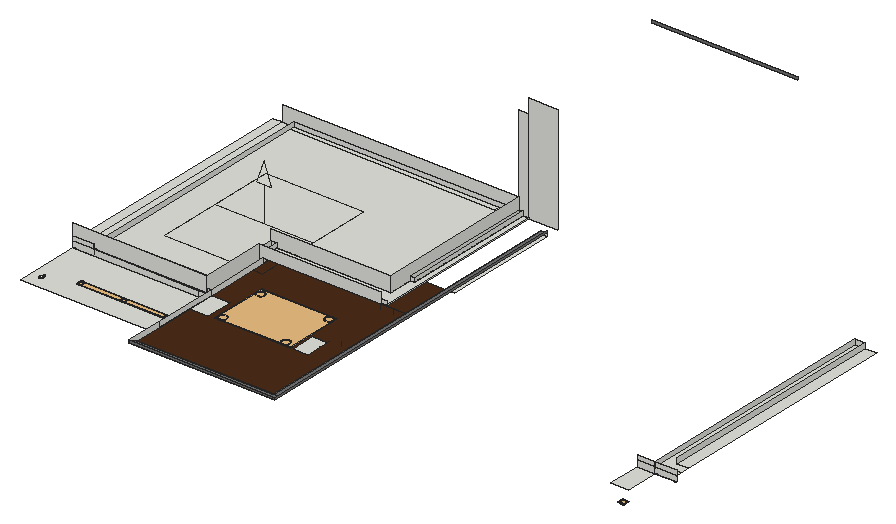
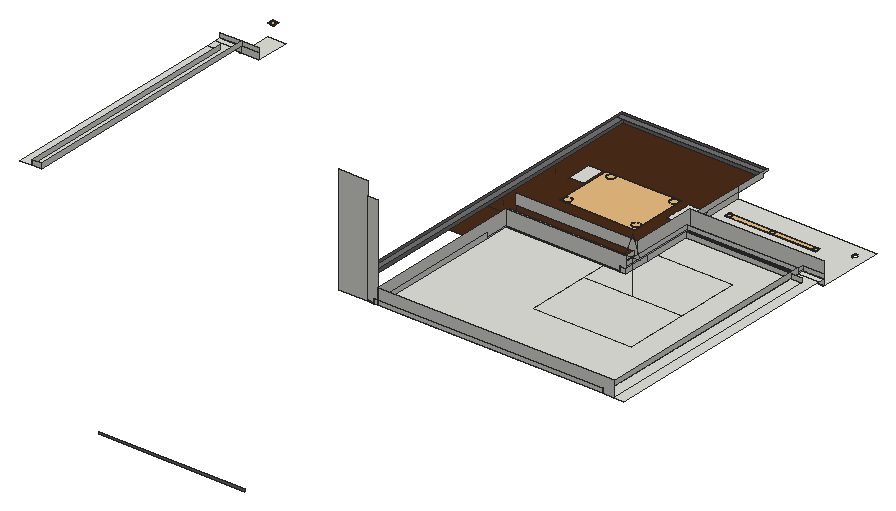
# SketchUp Ruby script. Lengths in inches.
U = 1.inch
M = Sketchup.active_model
def pt(a) = Geom::Point3d.new(a.map { |v| v * U })
def face(e, loops, mat)
  f = e.add_face(loops[0].map { |a| pt(a) })
  loops[1..].each { |l| e.add_face(l.map { |a| pt(a) }).erase! }
  f.material = f.back_material = mat if mat
  f
end
# faces: each face lists its corners as indices into pts; further lists are holes
def faces(e, pts, list, mat = nil) = list.each { |f| face(e, (f[0].is_a?(Array) ? f : [f]).map { |l| l.map { |i| pts[i] } }, mat) }
# xy, xz, yz: faces in a plane at the given z, y or x. An outline is a flat list of corners, or four numbers for a rectangle; further outlines are holes
def ring(l) = l.size == 4 ? [[l[0], l[1]], [l[2], l[1]], [l[2], l[3]], [l[0], l[3]]] : l.each_slice(2).to_a
def flat(e, list, mat, &to3) = list.each { |f| face(e, (f[0].is_a?(Array) ? f : [f]).map { |l| ring(l).map { |u, v| to3.(u, v) } }, mat) }
def xy(e, z, list, mat = nil) = flat(e, list, mat) { |x, y| [x, y, z] }
def xz(e, y, list, mat = nil) = flat(e, list, mat) { |x, z| [x, y, z] }
def yz(e, x, list, mat = nil) = flat(e, list, mat) { |y, z| [x, y, z] }
def lines(e, pts, list) = list.each { |a, b| e.add_line(pt(pts[a]), pt(pts[b])) }
# prism: a flat outline (further loops are holes) pulled along v
def prism(e, loops, v, mat = nil)
  f = face(e, loops, mat); d = Geom::Vector3d.new(v.map { |x| x * U })
  f.pushpull(f.normal.samedirection?(d) ? d.length : -d.length)
end
def box(e, o, s, mat = nil) = prism(e, [[o, [o[0] + s[0], o[1], o[2]], [o[0] + s[0], o[1] + s[1], o[2]], [o[0], o[1] + s[1], o[2]]]], [0, 0, s[2]], mat)
def at(x, y, z, deg = 0) = Geom::Transformation.translation(pt([x, y, z])) * Geom::Transformation.rotation(ORIGIN, Z_AXIS, deg.degrees)
def axes(o, x, y, z) = Geom::Transformation.new([*x, 0, *y, 0, *z, 0, *pt(o).to_a, 1])
def part(name) = M.definitions.add(name)
# library, detail: a bought-in or finely detailed component or shape, given as its bounding box
def library(name, o, s) = part(name).tap { |d| box(d.entities, o, s) }
def detail(e, o, s) = box(e.add_group.entities, o, s)
def put(e, d, t, mat = nil) = e.add_instance(d, t).tap { |i| i.material = mat if mat }
def group(e, t, mat = nil) = e.add_group.tap { |g| g.transformation = t; g.material = mat if mat }.entities
root = M.entities
M.materials.add("[Color M05]").color = [114, 114, 114]
M.materials.add("[Wood Veneer 01]").color = [76, 44, 23]
c1 = library("Group\#26",[-0.5,-0.5,-0.1],[9.125,9.125,0.2])
c2 = library("Group\#20",[-0.5,-0.5,-0.1],[139.5,7.875,0.2])
c3 = library("Group\#21",[-0.5,-0.5,-0.1],[115.36,88.99,0.2])
c4 = part("Group266\#1")
p = [[0,0,0],[0,0,-53.16],[-11.52,0,-53.16],[75.01,-97.09,0],[-75.01,-97.09,0],[75.01,97.09,0],
  [75.01,0,0],[-75.01,97.09,0],[11.52,0,-53.16],[-75.01,0,0],[0,0,-86.05]]
lines(c4.entities,p,[[0,1],[1,2],[3,4],[5,6],[7,5],[1,8],[9,0],[0,6],[8,10],[4,9],[6,3],[2,10],
  [9,7]])
c5 = part("Rectangle Light\#1")
put(c5.entities,c4,at(0,0,0))
xy(root,104.9375,[[[1172.33,538.49,1384.3,638.99],[1186.89,556.14,1187.94,556.28,1188.92,556.69,1189.77,557.33,1190.41,558.17,1190.82,559.15,1190.96,560.2,1190.82,561.26,1190.41,562.23,1189.77,563.08,1188.92,563.72,1187.94,564.13,1186.89,564.27,1185.84,564.13,1184.86,563.72,1184.02,563.08,1183.375,562.23,1182.97,561.26,1182.83,560.2,1182.97,559.15,1183.375,558.17,1184.02,557.33,1184.86,556.69,1185.84,556.28],[1234.95,572.82,1235.84,572.9375,1236.67,573.28,1237.38,573.83,1237.93,574.54,1238.27,575.37,1238.39,576.26,1238.27,577.15,1237.93,577.98,1237.38,578.6875,1236.67,579.23,1235.84,579.58,1234.95,579.69,1234.06,579.58,1233.23,579.23,1232.52,578.6875,1231.97,577.98,1231.63,577.15,1231.51,576.26,1231.63,575.37,1231.97,574.54,1232.52,573.83,1233.23,573.28,1234.06,572.9375],[1300.76,572.82,1301.65,572.9375,1302.48,573.28,1303.19,573.83,1303.74,574.54,1304.08,575.37,1304.2,576.26,1304.08,577.15,1303.74,577.98,1303.19,578.6875,1302.48,579.23,1301.65,579.58,1300.76,579.69,1299.87,579.58,1299.04,579.23,1298.33,578.6875,1297.79,577.98,1297.44,577.15,1297.32,576.26,1297.44,575.37,1297.79,574.54,1298.33,573.83,1299.04,573.28,1299.87,572.9375],[1366.57,572.82,1367.46,572.9375,1368.29,573.28,1369.01,573.83,1369.55,574.54,1369.9,575.37,1370.01,576.26,1369.9,577.15,1369.55,577.98,1369.01,578.6875,1368.29,579.23,1367.46,579.58,1366.57,579.69,1365.69,579.58,1364.86,579.23,1364.14,578.6875,1363.6,577.98,1363.25,577.15,1363.14,576.26,1363.25,575.37,1363.6,574.54,1364.14,573.83,1364.86,573.28,1365.69,572.9375]]])
xy(root,109.5,[[2037.92,586.4375,2064.92,636.6875]])
xy(root,113.8125,[[1384.3,597.99,1411.73,638.93],[1542.45,597.99,1563.95,635.56],[1172.33,638.99,1204.64,648.22],[1204.64,638.99,1365.47,648.22],[1172.33,648.22,1204.64,648.22,1204.64,662.52,1187.0625,662.52,1187.0625,1021.31,1172.33,1021.31],
  [1187.0625,662.52,1204.64,1021.31],[1204.64,662.52,1204.64,1013.93,1548.25,1013.93,1548.25,776.62,1364.27,776.62,1364.27,662.52],[1554.73,749.87,1563.95,1021.31],[1597.39,824.85,1607.7,1001.66],[1204.64,1013.93,1517.39,1021.31],
  [1517.39,1013.93,1548.25,1021.31]])
xy(root,113.8125,[[[1384.3,491.12,1384.3,597.99,1411.73,597.99,1411.73,638.93,1384.3,638.93,1384.3,749.87,1597.39,749.87,1597.39,491.12],[1542.45,597.99,1563.95,635.56],[1525.93,598.1875,1527.48,598.39,1528.93,598.99,1530.17,599.94,1531.13,601.1875,1531.73,602.63,1531.93,604.1875,1531.73,605.74,1531.13,607.1875,1530.17,608.43,1528.93,609.38,1527.48,609.98,1525.93,610.1875,1524.38,609.98,1522.93,609.38,1521.6875,608.43,1520.74,607.1875,1520.14,605.74,1519.93,604.1875,1520.14,602.63,1520.74,601.1875,1521.6875,599.94,1522.93,598.99,1524.38,598.39],[1429.12,670.9375,1430.67,671.14,1432.12,671.74,1433.36,672.69,1434.32,673.9375,1434.92,675.38,1435.12,676.9375,1434.92,678.49,1434.32,679.9375,1433.36,681.18,1432.12,682.13,1430.67,682.73,1429.12,682.9375,1427.57,682.73,1426.12,682.13,1424.875,681.18,1423.92,679.9375,1423.32,678.49,1423.12,676.9375,1423.32,675.38,1423.92,673.9375,1424.875,672.69,1426.12,671.74,1427.57,671.14],[1429.12,598.1875,1430.67,598.39,1432.12,598.99,1433.36,599.94,1434.32,601.1875,1434.92,602.63,1435.12,604.1875,1434.92,605.74,1434.32,607.1875,1433.36,608.43,1432.12,609.38,1430.67,609.98,1429.12,610.1875,1427.57,609.98,1426.12,609.38,1424.875,608.43,1423.92,607.1875,1423.32,605.74,1423.12,604.1875,1423.32,602.63,1423.92,601.1875,1424.875,599.94,1426.12,598.99,1427.57,598.39],[1531.48,674.17,1533.03,674.38,1534.48,674.98,1535.72,675.93,1536.68,677.17,1537.28,678.62,1537.48,680.17,1537.28,681.73,1536.68,683.17,1535.72,684.42,1534.48,685.37,1533.03,685.97,1531.48,686.17,1529.93,685.97,1528.48,685.37,1527.24,684.42,1526.28,683.17,1525.6875,681.73,1525.48,680.17,1525.6875,678.62,1526.28,677.17,1527.24,675.93,1528.48,674.98,1529.93,674.38]],[1563.95,749.87,1597.39,824.85]],"[Wood Veneer 01]")
xy(root,115.0625,[[1204.64,638.99,1376.89,638.99,1376.89,738.06,1384.3,738.06,1384.3,749.87,1563.95,749.87,1563.95,1021.31,1554.73,1021.31,1554.73,813.85,1548.25,813.85,1548.25,776.62,1373.95,776.62,1373.95,648.22,1204.64,648.22]])
xy(root,118.1875,[[1384.3,481.81,1607.7,491.12],[1597.39,491.12,1607.7,1001.66]],"[Color M05]")
xy(root,118.5,[[2064.92,636.6875,2097.23,645.91],[2064.92,645.91,2097.23,645.91,2097.23,660.21,2079.65,660.21,2079.65,1019,2064.92,1019],[2079.65,660.21,2097.23,1019]])
xz(root,481.81,[[1384.3,118.1875,1607.7,121.3125]],"[Color M05]")
xz(root,491.12,[[1384.3,113.8125,1597.39,118.1875]],"[Color M05]")
xz(root,636.6875,[[2037.92,109.5,2064.92,118.5],[2064.92,109.5,2097.23,109.625],[2064.92,109.625,2097.23,118.5],[2037.92,118.5,2064.92,126],[2064.92,118.5,2097.23,126]])
xz(root,638.99,[[1172.33,104.8125,1204.64,104.9375],[1172.33,104.9375,1204.64,113.8125],[1204.64,104.9375,1365.47,113.8125],[1365.47,104.9375,1384.3,113.8125],[1172.33,113.8125,1204.64,121.3125],
  [1204.64,113.8125,1376.89,115.0625],[1376.89,113.8125,1384.3,121.3125],[1204.64,115.0625,1376.89,115.0625,1376.89,138.1875,1172.33,138.1875,1172.33,121.3125,1204.64,121.3125]])
xz(root,648.22,[[1204.64,113.8125,1373.95,115.0625],[1204.64,115.0625,1373.95,121.3125]])
xz(root,662.52,[[1187.0625,113.8125,1364.27,121.3125]])
xz(root,738.06,[[1376.89,113.8125,1384.3,115.0625],[1376.89,115.0625,1384.3,115.0625,1384.3,121.3125,1563.95,121.3125,1563.95,138.1875,1376.89,138.1875]])
xz(root,749.87,[[1384.3,113.8125,1554.73,115.0625],[1554.73,113.8125,1563.95,115.0625],[1384.3,115.0625,1563.95,121.3125]])
xz(root,776.62,[[1364.27,113.8125,1373.95,121.3125],[1373.95,113.8125,1548.25,115.0625],[1373.95,115.0625,1548.25,115.0625,1548.25,138.1875,1364.27,138.1875,1364.27,121.3125,1373.95,121.3125]])
xz(root,813.85,[[1548.25,113.8125,1554.73,115.0625],[1548.25,115.0625,1554.73,121.3125]])
xz(root,1001.66,[[1597.39,113.8125,1607.7,118.1875]])
xz(root,1019,[[2064.92,118.5,2079.65,126]])
xz(root,1021.31,[[1187.0625,113.8125,1187.0625,138.1875,1548.25,138.1875,1548.25,121.3125,1204.64,121.3125,1204.64,113.8125],[1204.64,113.8125,1548.25,121.3125],[1548.25,113.8125,1554.73,121.3125],[1554.73,113.8125,1563.95,115.0625],[1563.95,113.8125,1607.7,279.25],
  [1554.73,115.0625,1554.73,121.3125,1548.25,121.3125,1548.25,258.1875,1563.95,258.1875,1563.95,115.0625]])
xz(root,1481.16,[[1384.3,118.1875,1607.7,121.3125]],"[Color M05]")
yz(root,1204.64,[[638.99,113.8125,648.22,115.0625],[648.22,113.8125,1021.31,121.3125],[638.99,115.0625,648.22,121.3125]])
yz(root,1364.27,[[662.52,113.8125,738.06,121.3125],[738.06,113.8125,776.62,121.3125]])
yz(root,1373.95,[[648.22,113.8125,776.62,115.0625],[648.22,115.0625,776.62,121.3125]])
yz(root,1376.89,[[638.99,113.8125,738.06,115.0625],[638.99,115.0625,738.06,138.1875]])
yz(root,1384.3,[[538.49,104.9375,597.99,113.8125],[597.99,104.9375,638.93,113.8125],[638.93,104.9375,638.99,113.8125],[491.12,113.8125,491.12,118.1875,481.81,118.1875,481.81,121.3125,538.49,121.3125,538.49,113.8125],[538.49,113.8125,638.99,121.3125],
  [638.99,113.8125,738.06,121.3125],[738.06,113.8125,749.87,115.0625],[738.06,115.0625,749.87,121.3125]])
yz(root,1548.25,[[776.62,113.8125,813.85,115.0625],[813.85,113.8125,1021.31,121.3125],[776.62,115.0625,813.85,115.0625,813.85,121.3125,1021.31,121.3125,1021.31,138.1875,776.62,138.1875]])
yz(root,1554.73,[[813.85,113.8125,1021.31,115.0625],[813.85,115.0625,1021.31,121.3125]])
yz(root,1563.95,[[749.87,113.8125,1021.31,115.0625]])
yz(root,1597.39,[[491.12,113.8125,1001.66,118.1875]],"[Color M05]")
yz(root,1607.7,[[481.81,118.1875,1001.66,121.3125]],"[Color M05]")
yz(root,2064.92,[[636.6875,118.5,1019,126]])
yz(root,2079.65,[[660.21,118.5,1019,126]])
p = [[1187.94,556.28,104.9375],[1186.89,556.14,104.9375],[1186.89,556.14,105.875],[1187.94,556.28,105.875],[1188.92,556.69,104.9375],[1188.92,556.69,105.875],
  [1189.77,557.33,104.9375],[1189.77,557.33,105.875],[1190.41,558.17,104.9375],[1190.41,558.17,105.875],[1190.82,559.15,104.9375],[1190.82,559.15,105.875],
  [1190.96,560.2,104.9375],[1190.96,560.2,105.875],[1190.82,561.26,104.9375],[1190.82,561.26,105.875],[1190.41,562.23,104.9375],[1190.41,562.23,105.875],
  [1189.77,563.08,104.9375],[1189.77,563.08,105.875],[1188.92,563.72,104.9375],[1188.92,563.72,105.875],[1187.94,564.13,104.9375],[1187.94,564.13,105.875],
  [1186.89,564.27,104.9375],[1186.89,564.27,105.875],[1234.95,572.82,104.9375],[1234.06,572.9375,104.9375],[1234.06,572.9375,105.375],[1234.95,572.82,105.375],
  [1235.84,572.9375,104.9375],[1235.84,572.9375,105.375],[1300.76,572.82,104.9375],[1299.87,572.9375,104.9375],[1299.87,572.9375,105.375],[1300.76,572.82,105.375],
  [1301.65,572.9375,104.9375],[1301.65,572.9375,105.375],[1366.57,572.82,104.9375],[1365.69,572.9375,104.9375],[1365.69,572.9375,105.375],[1366.57,572.82,105.375],
  [1367.46,572.9375,104.9375],[1367.46,572.9375,105.375],[1233.23,573.28,104.9375],[1233.23,573.28,105.375],[1236.67,573.28,104.9375],[1236.67,573.28,105.375],
  [1299.04,573.28,104.9375],[1299.04,573.28,105.375],[1302.48,573.28,104.9375],[1302.48,573.28,105.375],[1364.86,573.28,104.9375],[1364.86,573.28,105.375],
  [1368.29,573.28,104.9375],[1368.29,573.28,105.375],[1232.52,573.83,104.9375],[1232.52,573.83,105.375],[1237.38,573.83,104.9375],[1237.38,573.83,105.375],
  [1298.33,573.83,104.9375],[1298.33,573.83,105.375],[1303.19,573.83,104.9375],[1303.19,573.83,105.375],[1364.14,573.83,104.9375],[1364.14,573.83,105.375],
  [1369.01,573.83,104.9375],[1369.01,573.83,105.375],[1231.97,574.54,104.9375],[1231.97,574.54,105.375],[1237.93,574.54,104.9375],[1237.93,574.54,105.375],
  [1297.79,574.54,104.9375],[1297.79,574.54,105.375],[1303.74,574.54,104.9375],[1303.74,574.54,105.375],[1363.6,574.54,104.9375],[1363.6,574.54,105.375],
  [1369.55,574.54,104.9375],[1369.55,574.54,105.375],[1231.63,575.37,104.9375],[1231.63,575.37,105.375],[1238.27,575.37,104.9375],[1238.27,575.37,105.375],
  [1297.44,575.37,104.9375],[1297.44,575.37,105.375],[1304.08,575.37,104.9375],[1304.08,575.37,105.375],[1363.25,575.37,104.9375],[1363.25,575.37,105.375],
  [1369.9,575.37,104.9375],[1369.9,575.37,105.375],[1231.51,576.26,104.9375],[1231.51,576.26,105.375],[1238.39,576.26,104.9375],[1238.39,576.26,105.375],
  [1297.32,576.26,104.9375],[1297.32,576.26,105.375],[1304.2,576.26,104.9375],[1304.2,576.26,105.375],[1363.14,576.26,104.9375],[1363.14,576.26,105.375],
  [1370.01,576.26,104.9375],[1370.01,576.26,105.375],[1231.63,577.15,104.9375],[1231.63,577.15,105.375],[1238.27,577.15,104.9375],[1238.27,577.15,105.375],
  [1297.44,577.15,104.9375],[1297.44,577.15,105.375],[1304.08,577.15,104.9375],[1304.08,577.15,105.375],[1363.25,577.15,104.9375],[1363.25,577.15,105.375],
  [1369.9,577.15,104.9375],[1369.9,577.15,105.375],[1231.97,577.98,104.9375],[1231.97,577.98,105.375],[1237.93,577.98,104.9375],[1237.93,577.98,105.375],
  [1297.79,577.98,104.9375],[1297.79,577.98,105.375],[1303.74,577.98,104.9375],[1303.74,577.98,105.375],[1363.6,577.98,104.9375],[1363.6,577.98,105.375],
  [1369.55,577.98,104.9375],[1369.55,577.98,105.375],[1232.52,578.6875,104.9375],[1232.52,578.6875,105.375],[1237.38,578.6875,104.9375],[1237.38,578.6875,105.375],
  [1298.33,578.6875,104.9375],[1298.33,578.6875,105.375],[1303.19,578.6875,104.9375],[1303.19,578.6875,105.375],[1364.14,578.6875,104.9375],[1364.14,578.6875,105.375],
  [1369.01,578.6875,104.9375],[1369.01,578.6875,105.375],[1233.23,579.23,104.9375],[1233.23,579.23,105.375],[1236.67,579.23,104.9375],[1236.67,579.23,105.375],
  [1299.04,579.23,104.9375],[1299.04,579.23,105.375],[1302.48,579.23,104.9375],[1302.48,579.23,105.375],[1364.86,579.23,104.9375],[1364.86,579.23,105.375],
  [1368.29,579.23,104.9375],[1368.29,579.23,105.375],[1234.06,579.58,104.9375],[1234.06,579.58,105.375],[1235.84,579.58,104.9375],[1235.84,579.58,105.375],
  [1299.87,579.58,104.9375],[1299.87,579.58,105.375],[1301.65,579.58,104.9375],[1301.65,579.58,105.375],[1365.69,579.58,104.9375],[1365.69,579.58,105.375],
  [1367.46,579.58,104.9375],[1367.46,579.58,105.375],[1234.95,579.69,104.9375],[1234.95,579.69,105.375],[1300.76,579.69,104.9375],[1300.76,579.69,105.375],
  [1366.57,579.69,104.9375],[1366.57,579.69,105.375],[2079.48,553.83,109.625],[2078.43,553.97,109.625],[2078.43,553.97,110.5625],[2079.48,553.83,110.5625],
  [2080.53,553.97,109.625],[2080.53,553.97,110.5625],[2077.45,554.38,109.625],[2077.45,554.38,110.5625],[2081.51,554.38,109.625],[2081.51,554.38,110.5625],
  [2076.61,555.02,109.625],[2076.61,555.02,110.5625],[2082.36,555.02,109.625],[2082.36,555.02,110.5625],[2075.96,555.87,109.625],[2075.96,555.87,110.5625],
  [2083,555.87,109.625],[2083,555.87,110.5625],[2075.56,556.85,109.625],[2075.56,556.85,110.5625],[2083.41,556.85,109.625],[2083.41,556.85,110.5625],
  [2075.42,557.9,109.625],[2075.42,557.9,110.5625],[2083.55,557.9,109.625],[2083.55,557.9,110.5625],[2075.56,558.95,109.625],[2075.56,558.95,110.5625],
  [2083.41,558.95,109.625],[2083.41,558.95,110.5625],[2075.96,559.93,109.625],[2075.96,559.93,110.5625],[2083,559.93,109.625],[2083,559.93,110.5625],
  [2076.61,560.77,109.625],[2076.61,560.77,110.5625],[2082.36,560.77,109.625],[2082.36,560.77,110.5625],[2077.45,561.42,109.625],[2077.45,561.42,110.5625],
  [2081.51,561.42,109.625],[2081.51,561.42,110.5625],[2078.43,561.82,109.625],[2078.43,561.82,110.5625],[2080.53,561.82,109.625],[2080.53,561.82,110.5625],
  [2079.48,561.96,109.625],[2079.48,561.96,110.5625],[1429.12,598.1875,113.8125],[1427.57,598.39,113.8125],[1427.57,598.39,114.6875],[1429.12,598.1875,114.6875],
  [1430.67,598.39,113.8125],[1430.67,598.39,114.6875],[1525.93,598.1875,113.8125],[1524.38,598.39,113.8125],[1524.38,598.39,114.6875],[1525.93,598.1875,114.6875],
  [1527.48,598.39,113.8125],[1527.48,598.39,114.6875],[1426.12,598.99,113.8125],[1426.12,598.99,114.6875],[1432.12,598.99,113.8125],[1432.12,598.99,114.6875],
  [1522.93,598.99,113.8125],[1522.93,598.99,114.6875],[1528.93,598.99,113.8125],[1528.93,598.99,114.6875],[1424.875,599.94,113.8125],[1424.875,599.94,114.6875],
  [1433.36,599.94,113.8125],[1433.36,599.94,114.6875],[1521.6875,599.94,113.8125],[1521.6875,599.94,114.6875],[1530.17,599.94,113.8125],[1530.17,599.94,114.6875],
  [1423.92,601.1875,113.8125],[1423.92,601.1875,114.6875],[1434.32,601.1875,113.8125],[1434.32,601.1875,114.6875],[1520.74,601.1875,113.8125],[1520.74,601.1875,114.6875],
  [1531.13,601.1875,113.8125],[1531.13,601.1875,114.6875],[1423.32,602.63,113.8125],[1423.32,602.63,114.6875],[1434.92,602.63,113.8125],[1434.92,602.63,114.6875],
  [1520.14,602.63,113.8125],[1520.14,602.63,114.6875],[1531.73,602.63,113.8125],[1531.73,602.63,114.6875],[1423.12,604.1875,113.8125],[1423.12,604.1875,114.6875],
  [1435.12,604.1875,113.8125],[1435.12,604.1875,114.6875],[1519.93,604.1875,113.8125],[1519.93,604.1875,114.6875],[1531.93,604.1875,113.8125],[1531.93,604.1875,114.6875],
  [1423.32,605.74,113.8125],[1423.32,605.74,114.6875],[1434.92,605.74,113.8125],[1434.92,605.74,114.6875],[1520.14,605.74,113.8125],[1520.14,605.74,114.6875],
  [1531.73,605.74,113.8125],[1531.73,605.74,114.6875],[1423.92,607.1875,113.8125],[1423.92,607.1875,114.6875],[1434.32,607.1875,113.8125],[1434.32,607.1875,114.6875],
  [1520.74,607.1875,113.8125],[1520.74,607.1875,114.6875],[1531.13,607.1875,113.8125],[1531.13,607.1875,114.6875],[1424.875,608.43,113.8125],[1424.875,608.43,114.6875],
  [1433.36,608.43,113.8125],[1433.36,608.43,114.6875],[1521.6875,608.43,113.8125],[1521.6875,608.43,114.6875],[1530.17,608.43,113.8125],[1530.17,608.43,114.6875],
  [1426.12,609.38,113.8125],[1426.12,609.38,114.6875],[1432.12,609.38,113.8125],[1432.12,609.38,114.6875],[1522.93,609.38,113.8125],[1522.93,609.38,114.6875],
  [1528.93,609.38,113.8125],[1528.93,609.38,114.6875],[1427.57,609.98,113.8125],[1427.57,609.98,114.6875],[1430.67,609.98,113.8125],[1430.67,609.98,114.6875],
  [1524.38,609.98,113.8125],[1524.38,609.98,114.6875],[1527.48,609.98,113.8125],[1527.48,609.98,114.6875],[1429.12,610.1875,113.8125],[1429.12,610.1875,114.6875],
  [1525.93,610.1875,113.8125],[1525.93,610.1875,114.6875],[1429.12,670.9375,113.8125],[1427.57,671.14,113.8125],[1427.57,671.14,114.6875],[1429.12,670.9375,114.6875],
  [1430.67,671.14,113.8125],[1430.67,671.14,114.6875],[1426.12,671.74,113.8125],[1426.12,671.74,114.6875],[1432.12,671.74,113.8125],[1432.12,671.74,114.6875],
  [1424.875,672.69,113.8125],[1424.875,672.69,114.6875],[1433.36,672.69,113.8125],[1433.36,672.69,114.6875],[1423.92,673.9375,113.8125],[1423.92,673.9375,114.6875],
  [1434.32,673.9375,113.8125],[1434.32,673.9375,114.6875],[1423.32,675.38,113.8125],[1423.32,675.38,114.6875],[1434.92,675.38,113.8125],[1434.92,675.38,114.6875],
  [1531.48,674.17,113.8125],[1529.93,674.38,113.8125],[1529.93,674.38,114.6875],[1531.48,674.17,114.6875],[1533.03,674.38,113.8125],[1533.03,674.38,114.6875],
  [1528.48,674.98,113.8125],[1528.48,674.98,114.6875],[1534.48,674.98,113.8125],[1534.48,674.98,114.6875],[1527.24,675.93,113.8125],[1527.24,675.93,114.6875],
  [1535.72,675.93,113.8125],[1535.72,675.93,114.6875],[1423.12,676.9375,113.8125],[1423.12,676.9375,114.6875],[1435.12,676.9375,113.8125],[1435.12,676.9375,114.6875],
  [1526.28,677.17,113.8125],[1526.28,677.17,114.6875],[1536.68,677.17,113.8125],[1536.68,677.17,114.6875],[1423.32,678.49,113.8125],[1423.32,678.49,114.6875],
  [1434.92,678.49,113.8125],[1434.92,678.49,114.6875],[1525.6875,678.62,113.8125],[1525.6875,678.62,114.6875],[1537.28,678.62,113.8125],[1537.28,678.62,114.6875],
  [1423.92,679.9375,113.8125],[1423.92,679.9375,114.6875],[1434.32,679.9375,113.8125],[1434.32,679.9375,114.6875],[1525.48,680.17,113.8125],[1525.48,680.17,114.6875],
  [1537.48,680.17,113.8125],[1537.48,680.17,114.6875],[1424.875,681.18,113.8125],[1424.875,681.18,114.6875],[1433.36,681.18,113.8125],[1433.36,681.18,114.6875],
  [1525.6875,681.73,113.8125],[1525.6875,681.73,114.6875],[1537.28,681.73,113.8125],[1537.28,681.73,114.6875],[1426.12,682.13,113.8125],[1426.12,682.13,114.6875],
  [1432.12,682.13,113.8125],[1432.12,682.13,114.6875],[1526.28,683.17,113.8125],[1526.28,683.17,114.6875],[1536.68,683.17,113.8125],[1536.68,683.17,114.6875],
  [1427.57,682.73,113.8125],[1427.57,682.73,114.6875],[1430.67,682.73,113.8125],[1430.67,682.73,114.6875],[1429.12,682.9375,113.8125],[1429.12,682.9375,114.6875],
  [1527.24,684.42,113.8125],[1527.24,684.42,114.6875],[1535.72,684.42,113.8125],[1535.72,684.42,114.6875],[1528.48,685.37,113.8125],[1528.48,685.37,114.6875],
  [1534.48,685.37,113.8125],[1534.48,685.37,114.6875],[1529.93,685.97,113.8125],[1529.93,685.97,114.6875],[1533.03,685.97,113.8125],[1533.03,685.97,114.6875],
  [1531.48,686.17,113.8125],[1531.48,686.17,114.6875],[1563.95,738.06,121.3125],[1563.95,738.06,113.8125],[1583.39,738.06,121.3125],[1583.39,738.06,113.8125],
  [1583.39,638.99,113.8125],[1583.39,638.93,113.8125],[1563.95,638.93,113.8125],[1563.95,635.56,113.8125],[1583.39,638.99,121.3125]]
faces(root,p,[[0,1,2,3],[4,0,3,5],[6,4,5,7],[8,6,7,9],[10,8,9,11],[12,10,11,13],[14,12,13,15],[16,14,15,17],
  [18,16,17,19],[20,18,19,21],[22,20,21,23],[24,22,23,25],[26,27,28,29],[30,26,29,31],[32,33,34,35],[36,32,35,37],
  [38,39,40,41],[42,38,41,43],[27,44,45,28],[46,30,31,47],[33,48,49,34],[50,36,37,51],[39,52,53,40],[54,42,43,55],
  [44,56,57,45],[58,46,47,59],[48,60,61,49],[62,50,51,63],[52,64,65,53],[66,54,55,67],[56,68,69,57],[70,58,59,71],
  [60,72,73,61],[74,62,63,75],[64,76,77,65],[78,66,67,79],[68,80,81,69],[82,70,71,83],[72,84,85,73],[86,74,75,87],
  [76,88,89,77],[90,78,79,91],[80,92,93,81],[94,82,83,95],[84,96,97,85],[98,86,87,99],[88,100,101,89],[102,90,91,103],
  [92,104,105,93],[106,94,95,107],[96,108,109,97],[110,98,99,111],[100,112,113,101],[114,102,103,115],[104,116,117,105],[118,106,107,119],
  [108,120,121,109],[122,110,111,123],[112,124,125,113],[126,114,115,127],[116,128,129,117],[130,118,119,131],[120,132,133,121],[134,122,123,135],
  [124,136,137,125],[138,126,127,139],[128,140,141,129],[142,130,131,143],[132,144,145,133],[146,134,135,147],[136,148,149,137],[150,138,139,151],
  [140,152,153,141],[154,142,143,155],[144,156,157,145],[158,146,147,159],[148,160,161,149],[162,150,151,163],[152,164,165,153],[164,154,155,165],
  [156,166,167,157],[166,158,159,167],[160,168,169,161],[168,162,163,169],[170,171,172,173],[174,170,173,175],[171,176,177,172],[178,174,175,179],
  [176,180,181,177],[182,178,179,183],[180,184,185,181],[186,182,183,187],[184,188,189,185],[190,186,187,191],[188,192,193,189],[194,190,191,195],
  [192,196,197,193],[198,194,195,199],[196,200,201,197],[202,198,199,203],[200,204,205,201],[206,202,203,207],[204,208,209,205],[210,206,207,211],
  [208,212,213,209],[214,210,211,215],[212,216,217,213],[216,214,215,217]])
faces(root,p,[[218,219,220,221],[222,218,221,223],[224,225,226,227],[228,224,227,229],[219,230,231,220],[232,222,223,233],[225,234,235,226],[236,228,229,237],
  [230,238,239,231],[240,232,233,241],[234,242,243,235],[244,236,237,245],[238,246,247,239],[248,240,241,249],[242,250,251,243],[252,244,245,253],
  [246,254,255,247],[256,248,249,257],[250,258,259,251],[260,252,253,261],[254,262,263,255],[264,256,257,265],[258,266,267,259],[268,260,261,269],
  [262,270,271,263],[272,264,265,273],[266,274,275,267],[276,268,269,277],[270,278,279,271],[280,272,273,281],[274,282,283,275],[284,276,277,285],
  [278,286,287,279],[288,280,281,289],[282,290,291,283],[292,284,285,293],[286,294,295,287],[296,288,289,297],[290,298,299,291],[300,292,293,301],
  [294,302,303,295],[304,296,297,305],[298,306,307,299],[308,300,301,309],[302,310,311,303],[310,304,305,311],[306,312,313,307],[312,308,309,313],
  [314,315,316,317],[318,314,317,319],[315,320,321,316],[322,318,319,323],[320,324,325,321],[326,322,323,327],[324,328,329,325],[330,326,327,331],
  [328,332,333,329],[334,330,331,335],[336,337,338,339],[340,336,339,341],[337,342,343,338],[344,340,341,345],[342,346,347,343],[348,344,345,349],
  [332,350,351,333],[352,334,335,353],[346,354,355,347],[356,348,349,357],[350,358,359,351],[360,352,353,361],[354,362,363,355],[364,356,357,365],
  [358,366,367,359],[368,360,361,369],[362,370,371,363],[372,364,365,373],[366,374,375,367],[376,368,369,377],[370,378,379,371],[380,372,373,381],
  [374,382,383,375],[384,376,377,385],[378,386,387,379],[388,380,381,389],[382,390,391,383],[392,384,385,393],[390,394,395,391],[394,392,393,395],
  [386,396,397,387],[398,388,389,399],[396,400,401,397],[402,398,399,403],[400,404,405,401],[406,402,403,407],[404,408,409,405],[408,406,407,409]],"[Wood Veneer 01]")
lines(root,p,[[410,411],[412,413],[414,415],[416,417],[414,418]])
put(root,c1,at(2075.42,553.83,110.5625))
put(root,c2,at(1231.51,572.82,105.375))
put(root,c3,at(1423.12,598.1875,114.6875))
put(root,c5,axes([1323.92,814.73,113.82],[1,0,0],[0,1,0],[0,0,-1]))
